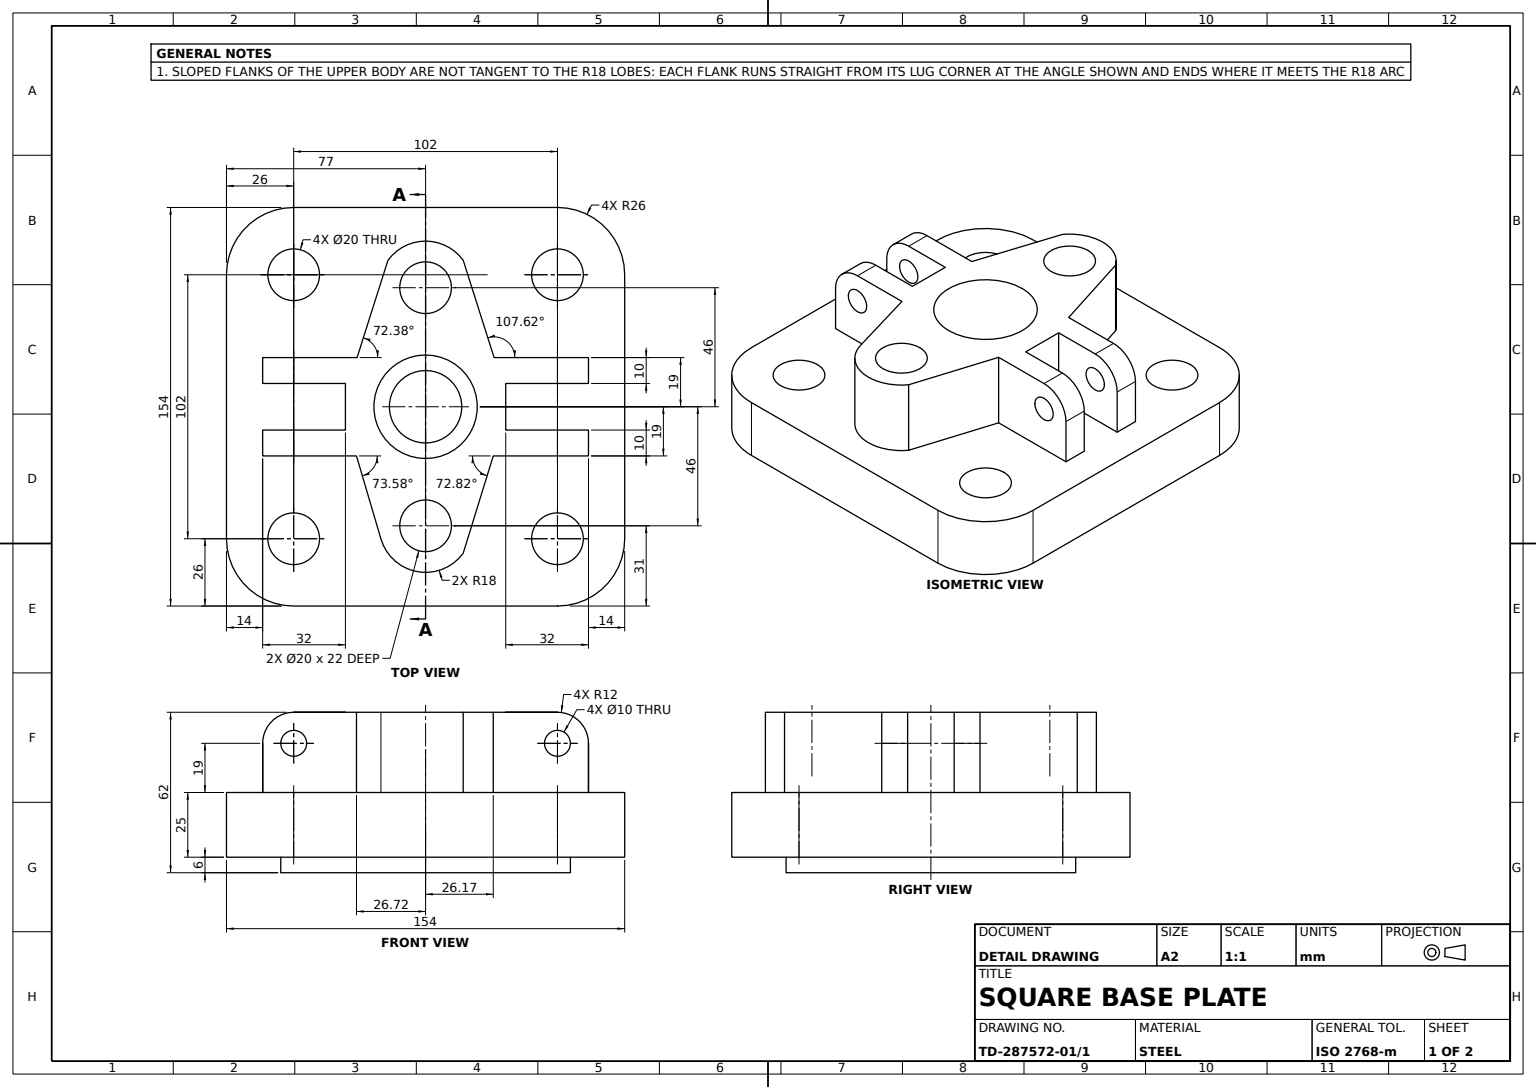
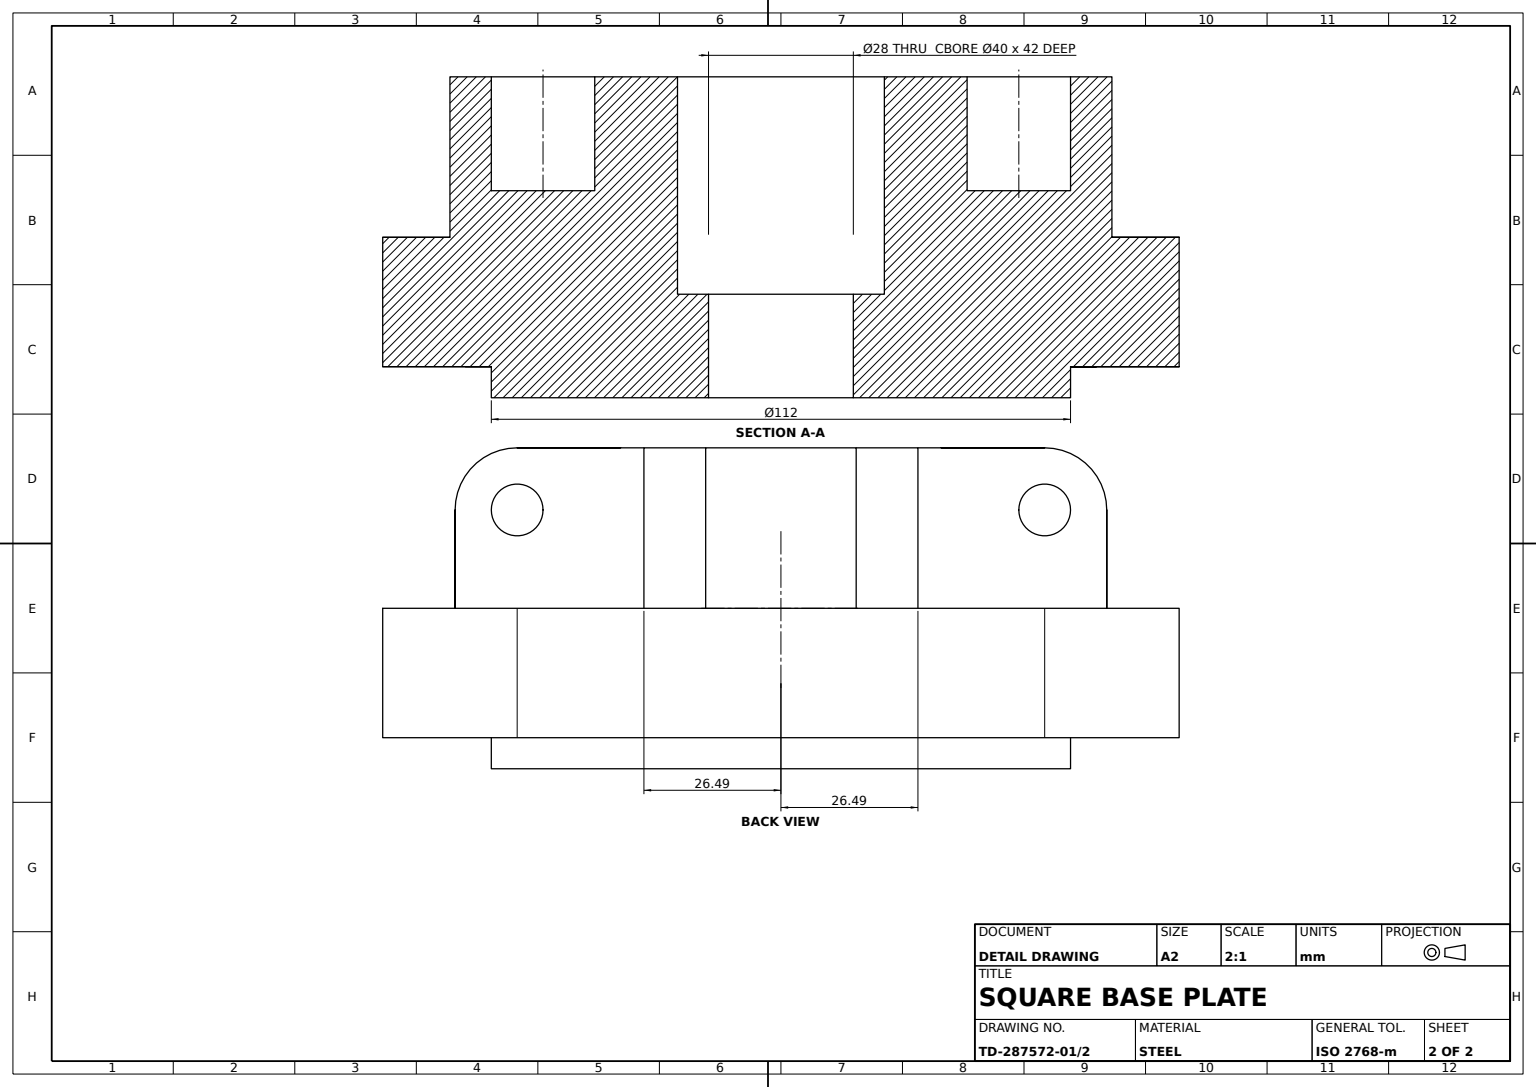
solid
v1 (-63,25,9)
v2 (-31,25,9)
e1 v1 v2 LINE
v3 (-63,44,9)
e2 v1 v3 LINE
v4 (-51,56,9)
e3 v3 v4 CIRCLE(AX(P(-51,44,9),D(0,0,-1),D(1,0,0)),12)
v5 (-31,56,9)
e4 v4 v5 LINE
e5 v2 v5 LINE
v6 (-46,44,9)
v7 (-56,44,9)
e6 v6 v7 CIRCLE(AX(P(-51,44,9),D(0,0,1),D(1,0,0)),5)
e7 v7 v6 CIRCLE(AX(P(-51,44,9),D(0,0,1),D(1,0,0)),5)
face PLANE(AX(P(0,25,9),D(0,0,1),D(1,0,0))) rev [-e1 e2 e3 e4 -e5] [e6 e7]
v8 (0,25,-64)
v9 (-14.551173,25,-56.595441)
e8 v8 v9 CIRCLE(AX(P(0,25,-46),D(0,1,0),D(0,0,1)),18)
v10 (-14.551173,56,-56.595441)
e9 v10 v9 LINE
v11 (0,56,-64)
e10 v11 v10 CIRCLE(AX(P(0,56,-46),D(0,1,0),D(0,0,1)),18)
e11 v11 v8 LINE
face CYL(AX(P(0,56,-46),D(0,-1,0),D(0,0,-1)),18) [e8 -e9 -e10 e11]
v12 (14.551173,56,56.595441)
v13 (14.551173,25,56.595441)
e12 v12 v13 LINE
v14 (-17.266235,56,51.086957)
e13 v14 v12 CIRCLE(AX(P(0,56,46),D(0,1,0),D(0,0,1)),18)
v15 (-17.266235,25,51.086957)
e14 v14 v15 LINE
e15 v15 v13 CIRCLE(AX(P(0,25,46),D(0,1,0),D(0,0,1)),18)
face CYL(AX(P(0,56,46),D(0,-1,0),D(0,0,-1)),18) [-e12 -e13 e14 e15]
v16 (-46,44,19)
v17 (-56,44,19)
e16 v16 v17 CIRCLE(AX(P(-51,44,19),D(0,0,1),D(1,0,0)),5)
e17 v7 v17 LINE
e18 v6 v16 LINE
face CYL(AX(P(-51,44,-99),D(0,0,1),D(1,0,0)),5) rev [e16 -e17 -e6 e18]
v18 (51,0,-61)
v19 (51,25,-61)
e19 v18 v19 LINE
v20 (51,25,-41)
e20 v19 v20 CIRCLE(AX(P(51,25,-51),D(0,1,0),D(0,0,1)),10)
v21 (51,0,-41)
e21 v21 v20 LINE
e22 v18 v21 CIRCLE(AX(P(51,0,-51),D(0,1,0),D(0,0,1)),10)
face CYL(AX(P(51,-87,-51),D(0,1,0),D(0,0,1)),10) rev [e19 e20 -e21 -e22]
v22 (63,44,9)
v23 (63,44,19)
e23 v22 v23 LINE
v24 (51,56,9)
e24 v24 v22 CIRCLE(AX(P(51,44,9),D(0,0,-1),D(-1,0,0)),12)
v25 (51,56,19)
e25 v25 v24 LINE
e26 v23 v25 CIRCLE(AX(P(51,44,19),D(0,0,1),D(1,0,0)),12)
face CYL(AX(P(51,44,-46),D(0,0,-1),D(-1,0,0)),12) [-e23 -e24 -e25 -e26]
v26 (-46,44,-19)
v27 (-56,44,-19)
e27 v26 v27 CIRCLE(AX(P(-51,44,-19),D(0,0,-1),D(-1,0,0)),5)
e28 v27 v26 CIRCLE(AX(P(-51,44,-19),D(0,0,-1),D(-1,0,0)),5)
v28 (-26.491517,25,-19)
v29 (-63,25,-19)
e29 v28 v29 LINE
v30 (-63,44,-19)
e30 v29 v30 LINE
v31 (-51,56,-19)
e31 v30 v31 CIRCLE(AX(P(-51,44,-19),D(0,0,-1),D(-1,0,0)),12)
v32 (-26.491517,56,-19)
e32 v32 v31 LINE
e33 v28 v32 LINE
face PLANE(AX(P(0,25,-19),D(0,0,-1),D(-1,0,0))) [-e27 -e28] [e29 e30 e31 -e32 -e33]
v33 (51,25,41)
v34 (51,25,61)
e34 v33 v34 CIRCLE(AX(P(51,25,51),D(0,1,0),D(0,0,1)),10)
v35 (51,0,61)
e35 v35 v34 LINE
v36 (51,0,41)
e36 v36 v35 CIRCLE(AX(P(51,0,51),D(0,1,0),D(0,0,1)),10)
e37 v36 v33 LINE
face CYL(AX(P(51,-87,51),D(0,1,0),D(0,0,1)),10) rev [e34 -e35 -e36 e37]
v37 (31,25,-9)
v38 (31,25,9)
e38 v37 v38 LINE
v39 (31,56,-9)
e39 v37 v39 LINE
v40 (31,56,9)
e40 v39 v40 LINE
e41 v38 v40 LINE
face PLANE(AX(P(31,25,0),D(-1,0,0),D(0,0,1))) rev [-e38 e39 e40 -e41]
v41 (-31,25,-9)
e42 v41 v2 LINE
v42 (-31,56,-9)
e43 v42 v5 LINE
e44 v41 v42 LINE
face PLANE(AX(P(-31,25,0),D(-1,0,0),D(0,0,1))) [e42 e5 -e43 -e44]
v43 (26.491517,25,-19)
v44 (63,25,-19)
e45 v43 v44 LINE
v45 (26.491517,56,-19)
e46 v43 v45 LINE
v46 (51,56,-19)
e47 v45 v46 LINE
v47 (63,44,-19)
e48 v46 v47 CIRCLE(AX(P(51,44,-19),D(0,0,-1),D(1,0,0)),12)
e49 v44 v47 LINE
v48 (46,44,-19)
v49 (56,44,-19)
e50 v48 v49 CIRCLE(AX(P(51,44,-19),D(0,0,1),D(1,0,0)),5)
e51 v49 v48 CIRCLE(AX(P(51,44,-19),D(0,0,1),D(1,0,0)),5)
face PLANE(AX(P(0,25,-19),D(0,0,1),D(1,0,0))) rev [-e45 e46 e47 e48 -e49] [e50 e51]
e52 v24 v40 LINE
v50 (63,25,9)
e53 v50 v22 LINE
e54 v50 v38 LINE
v51 (56,44,9)
v52 (46,44,9)
e55 v51 v52 CIRCLE(AX(P(51,44,9),D(0,0,-1),D(-1,0,0)),5)
e56 v52 v51 CIRCLE(AX(P(51,44,9),D(0,0,-1),D(-1,0,0)),5)
face PLANE(AX(P(0,25,9),D(0,0,-1),D(-1,0,0))) [-e52 e24 -e53 e54 e41] [-e55 -e56]
v53 (63,25,-9)
e57 v44 v53 LINE
v54 (63,44,-9)
e58 v47 v54 LINE
e59 v53 v54 LINE
face PLANE(AX(P(63,25,0),D(-1,0,0),D(0,0,1))) rev [-e57 e49 e58 -e59]
v55 (-46,44,-9)
e60 v26 v55 LINE
v56 (-56,44,-9)
e61 v55 v56 CIRCLE(AX(P(-51,44,-9),D(0,0,1),D(1,0,0)),5)
e62 v27 v56 LINE
face CYL(AX(P(-51,44,-99),D(0,0,1),D(1,0,0)),5) rev [e60 e61 -e62 e28]
v57 (77,0,-51)
v58 (51,0,-77)
e63 v57 v58 CIRCLE(AX(P(51,0,-51),D(0,1,0),D(0,0,1)),26)
v59 (77,0,51)
e64 v59 v57 LINE
v60 (51,0,77)
e65 v60 v59 CIRCLE(AX(P(51,0,51),D(0,1,0),D(0,0,1)),26)
v61 (-51,0,77)
e66 v61 v60 LINE
v62 (-77,0,51)
e67 v62 v61 CIRCLE(AX(P(-51,0,51),D(0,1,0),D(0,0,1)),26)
v63 (-77,0,-51)
e68 v63 v62 LINE
v64 (-51,0,-77)
e69 v64 v63 CIRCLE(AX(P(-51,0,-51),D(0,1,0),D(0,0,1)),26)
e70 v58 v64 LINE
e71 v35 v36 CIRCLE(AX(P(51,0,51),D(0,1,0),D(0,0,1)),10)
v65 (-51,0,41)
v66 (-51,0,61)
e72 v65 v66 CIRCLE(AX(P(-51,0,51),D(0,1,0),D(0,0,1)),10)
e73 v66 v65 CIRCLE(AX(P(-51,0,51),D(0,1,0),D(0,0,1)),10)
e74 v21 v18 CIRCLE(AX(P(51,0,-51),D(0,1,0),D(0,0,1)),10)
v67 (-51,0,-41)
v68 (-51,0,-61)
e75 v67 v68 CIRCLE(AX(P(-51,0,-51),D(0,1,0),D(0,0,1)),10)
e76 v68 v67 CIRCLE(AX(P(-51,0,-51),D(0,1,0),D(0,0,1)),10)
v69 (0,0,56)
v70 (0,0,-56)
e77 v69 v70 CIRCLE(AX(P(0,0,0),D(0,-1,0),D(0,0,-1)),56)
e78 v70 v69 CIRCLE(AX(P(0,0,0),D(0,-1,0),D(0,0,-1)),56)
face PLANE(AX(P(51,0,51),D(0,1,0),D(0,0,1))) rev [-e63 -e64 -e65 -e66 -e67 -e68 -e69 -e70] [e36 e71] [e72 e73] [e74 e22] [e75 e76] [-e77 -e78]
e79 v10 v32 LINE
e80 v9 v28 LINE
face PLANE(AX(P(-14.551173,56,-56.595441),D(0.953085629,0,0.302700815),D(0.302700815,0,-0.953085629))) rev [-e79 e9 e80 e33]
v71 (51,25,-77)
e81 v71 v58 LINE
v72 (77,25,-51)
e82 v72 v71 CIRCLE(AX(P(51,25,-51),D(0,1,0),D(0,0,1)),26)
e83 v72 v57 LINE
face CYL(AX(P(51,25,-51),D(0,-1,0),D(0,0,-1)),26) [-e81 -e82 e83 e63]
v73 (0,-6,14)
v74 (0,-6,-14)
e84 v73 v74 CIRCLE(AX(P(0,-6,0),D(0,-1,0),D(0,0,-1)),14)
v75 (0,14,-14)
e85 v74 v75 LINE
v76 (0,14,14)
e86 v76 v75 CIRCLE(AX(P(0,14,0),D(0,-1,0),D(0,0,1)),14)
e87 v73 v76 LINE
face CYL(AX(P(0,-62,0),D(0,1,0),D(0,0,1)),14) rev [e84 e85 -e86 -e87]
e88 v34 v33 CIRCLE(AX(P(51,25,51),D(0,1,0),D(0,0,1)),10)
face CYL(AX(P(51,-87,51),D(0,1,0),D(0,0,1)),10) rev [-e37 -e71 e35 e88]
v77 (-51,56,19)
e89 v4 v77 LINE
v78 (-63,44,19)
e90 v78 v3 LINE
e91 v77 v78 CIRCLE(AX(P(-51,44,19),D(0,0,1),D(-1,0,0)),12)
face CYL(AX(P(-51,44,0),D(0,0,1),D(1,0,0)),12) [-e89 -e3 -e90 -e91]
v79 (14.551173,56,-56.595441)
e92 v45 v79 LINE
v80 (14.551173,25,-56.595441)
e93 v43 v80 LINE
e94 v79 v80 LINE
face PLANE(AX(P(14.551173,56,-56.595441),D(-0.953085629,0,0.302700815),D(0.302700815,0,0.953085629))) rev [-e92 -e46 e93 -e94]
e95 v20 v19 CIRCLE(AX(P(51,25,-51),D(0,1,0),D(0,0,1)),10)
face CYL(AX(P(51,-87,-51),D(0,1,0),D(0,0,1)),10) rev [e21 e95 -e19 -e74]
v81 (0,-6,-56)
e96 v81 v70 LINE
v82 (0,-6,56)
e97 v82 v69 LINE
e98 v81 v82 CIRCLE(AX(P(0,-6,0),D(0,-1,0),D(0,0,-1)),56)
face CYL(AX(P(0,-6,0),D(0,1,0),D(0,0,1)),56) [e96 e78 -e97 -e98]
v83 (63,25,19)
e99 v83 v23 LINE
e100 v83 v50 LINE
face PLANE(AX(P(63,25,0),D(1,0,0),D(0,0,-1))) [-e99 e100 e53 e23]
v84 (-51,25,61)
v85 (-51,25,41)
e101 v84 v85 CIRCLE(AX(P(-51,25,51),D(0,1,0),D(0,0,1)),10)
e102 v65 v85 LINE
e103 v66 v84 LINE
face CYL(AX(P(-51,-87,51),D(0,1,0),D(0,0,1)),10) rev [e101 -e102 -e73 e103]
e104 v17 v16 CIRCLE(AX(P(-51,44,19),D(0,0,1),D(1,0,0)),5)
v86 (-63,25,19)
e105 v86 v78 LINE
v87 (-26.719654,25,19)
e106 v87 v86 LINE
v88 (-26.719654,56,19)
e107 v87 v88 LINE
e108 v88 v77 LINE
face PLANE(AX(P(0,25,19),D(0,0,-1),D(-1,0,0))) rev [-e16 -e104] [-e105 -e106 e107 e108 e91]
e109 v56 v55 CIRCLE(AX(P(-51,44,-9),D(0,0,1),D(1,0,0)),5)
face CYL(AX(P(-51,44,-99),D(0,0,1),D(1,0,0)),5) rev [-e60 e27 e62 e109]
e110 v88 v14 LINE
e111 v87 v15 LINE
face PLANE(AX(P(-29.736294,56,8.76087),D(0.959235281,0,-0.282608696),D(-0.282608696,0,-0.959235281))) rev [-e110 -e107 e111 -e14]
e112 v85 v84 CIRCLE(AX(P(-51,25,51),D(0,1,0),D(0,0,1)),10)
face CYL(AX(P(-51,-87,51),D(0,1,0),D(0,0,1)),10) rev [e112 -e103 -e72 e102]
v89 (0,14,-20)
v90 (0,14,20)
e113 v89 v90 CIRCLE(AX(P(0,14,0),D(0,1,0),D(0,0,1)),20)
v91 (0,56,-20)
e114 v89 v91 LINE
v92 (0,56,20)
e115 v91 v92 CIRCLE(AX(P(0,56,0),D(0,1,0),D(0,0,1)),20)
e116 v90 v92 LINE
face CYL(AX(P(0,14,0),D(0,1,0),D(0,0,1)),20) rev [-e113 e114 e115 -e116]
v93 (51,56,-9)
e117 v54 v93 CIRCLE(AX(P(51,44,-9),D(0,0,1),D(-1,0,0)),12)
e118 v93 v46 LINE
face CYL(AX(P(51,44,0),D(0,0,-1),D(-1,0,0)),12) [-e117 -e58 -e48 -e118]
v94 (0,56,-56)
v95 (0,56,-36)
e119 v94 v95 CIRCLE(AX(P(0,56,-46),D(0,1,0),D(0,0,1)),10)
v96 (0,34,-36)
e120 v96 v95 LINE
v97 (0,34,-56)
e121 v97 v96 CIRCLE(AX(P(0,34,-46),D(0,1,0),D(0,0,1)),10)
e122 v97 v94 LINE
face CYL(AX(P(0,34,-46),D(0,1,0),D(0,0,1)),10) rev [e119 -e120 -e121 e122]
v98 (46,44,19)
v99 (56,44,19)
e123 v98 v99 CIRCLE(AX(P(51,44,19),D(0,0,1),D(1,0,0)),5)
e124 v51 v99 LINE
e125 v52 v98 LINE
face CYL(AX(P(51,44,-99),D(0,0,1),D(1,0,0)),5) rev [e123 -e124 e55 e125]
e126 v92 v91 CIRCLE(AX(P(0,56,0),D(0,1,0),D(0,0,1)),20)
e127 v90 v89 CIRCLE(AX(P(0,14,0),D(0,1,0),D(0,0,1)),20)
face CYL(AX(P(0,14,0),D(0,1,0),D(0,0,1)),20) rev [e116 e126 -e114 -e127]
v100 (-51,56,-9)
e128 v31 v100 LINE
v101 (-63,44,-9)
e129 v101 v30 LINE
e130 v100 v101 CIRCLE(AX(P(-51,44,-9),D(0,0,1),D(1,0,0)),12)
face CYL(AX(P(-51,44,-46),D(0,0,1),D(1,0,0)),12) [-e128 -e31 -e129 -e130]
v102 (77,25,51)
e131 v102 v72 LINE
e132 v102 v59 LINE
face PLANE(AX(P(77,25,0),D(-1,0,0),D(0,0,1))) rev [e64 -e83 -e131 e132]
v103 (0,34,56)
v104 (0,56,56)
e133 v103 v104 LINE
v105 (0,34,36)
e134 v105 v103 CIRCLE(AX(P(0,34,46),D(0,1,0),D(0,0,1)),10)
v106 (0,56,36)
e135 v105 v106 LINE
e136 v106 v104 CIRCLE(AX(P(0,56,46),D(0,1,0),D(0,0,1)),10)
face CYL(AX(P(0,34,46),D(0,1,0),D(0,0,1)),10) rev [-e133 -e134 e135 e136]
e137 v80 v8 CIRCLE(AX(P(0,25,-46),D(0,1,0),D(0,0,1)),18)
e138 v79 v11 CIRCLE(AX(P(0,56,-46),D(0,1,0),D(0,0,1)),18)
face CYL(AX(P(0,56,-46),D(0,-1,0),D(0,0,-1)),18) [e137 -e11 -e138 e94]
v107 (-77,25,-51)
v108 (-77,25,51)
e139 v107 v108 LINE
e140 v107 v63 LINE
e141 v108 v62 LINE
face PLANE(AX(P(-77,25,-51),D(1,0,0),D(0,0,-1))) rev [-e139 e140 e68 -e141]
v109 (-51,25,-41)
e142 v67 v109 LINE
v110 (-51,25,-61)
e143 v109 v110 CIRCLE(AX(P(-51,25,-51),D(0,1,0),D(0,0,1)),10)
e144 v68 v110 LINE
face CYL(AX(P(-51,-87,-51),D(0,1,0),D(0,0,1)),10) rev [e142 e143 -e144 -e75]
e145 v96 v97 CIRCLE(AX(P(0,34,-46),D(0,1,0),D(0,0,1)),10)
face PLANE(AX(P(0,34,-46),D(0,1,0),D(0,0,1))) [e121 e145]
e146 v99 v98 CIRCLE(AX(P(51,44,19),D(0,0,1),D(1,0,0)),5)
face CYL(AX(P(51,44,-99),D(0,0,1),D(1,0,0)),5) rev [e56 e124 e146 -e125]
face CYL(AX(P(-51,44,-99),D(0,0,1),D(1,0,0)),5) rev [-e18 -e7 e17 e104]
v111 (-51,25,-77)
e147 v111 v64 LINE
e148 v71 v111 LINE
face PLANE(AX(P(51,25,-77),D(0,0,1),D(1,0,0))) rev [e70 -e147 -e148 e81]
e149 v111 v107 CIRCLE(AX(P(-51,25,-51),D(0,1,0),D(0,0,1)),26)
face CYL(AX(P(-51,25,-51),D(0,-1,0),D(0,0,-1)),26) [e69 -e140 -e149 e147]
v112 (46,44,-9)
e150 v48 v112 LINE
v113 (56,44,-9)
e151 v113 v112 CIRCLE(AX(P(51,44,-9),D(0,0,-1),D(-1,0,0)),5)
e152 v49 v113 LINE
face CYL(AX(P(51,44,-99),D(0,0,1),D(1,0,0)),5) rev [-e50 e150 -e151 -e152]
v114 (51,25,77)
e153 v114 v102 CIRCLE(AX(P(51,25,51),D(0,1,0),D(0,0,1)),26)
e154 v114 v60 LINE
face CYL(AX(P(51,25,51),D(0,-1,0),D(0,0,-1)),26) [-e153 e154 e65 -e132]
e155 v112 v113 CIRCLE(AX(P(51,44,-9),D(0,0,-1),D(-1,0,0)),5)
face CYL(AX(P(51,44,-99),D(0,0,1),D(1,0,0)),5) rev [-e150 -e51 e152 -e155]
e156 v95 v94 CIRCLE(AX(P(0,56,-46),D(0,1,0),D(0,0,1)),10)
face CYL(AX(P(0,34,-46),D(0,1,0),D(0,0,1)),10) rev [e156 -e122 -e145 e120]
e157 v86 v1 LINE
face PLANE(AX(P(-63,25,0),D(1,0,0),D(0,0,-1))) rev [e90 -e2 -e157 e105]
v115 (-63,25,-9)
e158 v29 v115 LINE
e159 v115 v101 LINE
face PLANE(AX(P(-63,25,0),D(-1,0,0),D(0,0,1))) [-e30 e158 e159 e129]
v116 (26.17373,56,19)
e160 v12 v116 LINE
e161 v116 v25 LINE
e162 v93 v39 LINE
e163 v100 v42 LINE
e164 v104 v106 CIRCLE(AX(P(0,56,46),D(0,1,0),D(0,0,1)),10)
face PLANE(AX(P(0,56,-46),D(0,1,0),D(0,0,1))) [e160 e161 e25 e52 -e40 -e162 e118 -e47 e92 e138 e10 e79 e32 e128 e163 e43 -e4 e89 -e108 e110 e13] [-e136 -e164] [-e126 -e115] [-e119 -e156]
v117 (-51,25,77)
e165 v108 v117 CIRCLE(AX(P(-51,25,51),D(0,1,0),D(0,0,1)),26)
e166 v117 v114 LINE
v118 (26.17373,25,19)
e167 v118 v83 LINE
e168 v13 v118 LINE
e169 v115 v41 LINE
e170 v53 v37 LINE
e171 v110 v109 CIRCLE(AX(P(-51,25,-51),D(0,1,0),D(0,0,1)),10)
face PLANE(AX(P(51,25,51),D(0,1,0),D(0,0,1))) [-e101 -e112] [-e95 -e20] [e82 e148 e149 e139 e165 e166 e153 e131] [-e54 -e100 -e167 -e168 -e15 -e111 e106 e157 e1 -e42 -e169 -e158 -e29 -e80 -e8 -e137 -e93 e45 e57 e170 e38] [-e143 -e171] [-e34 -e88]
e172 v118 v116 LINE
face PLANE(AX(P(0,25,19),D(0,0,1),D(1,0,0))) [-e161 -e172 e167 e99 e26] [-e146 -e123]
e173 v103 v105 CIRCLE(AX(P(0,34,46),D(0,1,0),D(0,0,1)),10)
face CYL(AX(P(0,34,46),D(0,1,0),D(0,0,1)),10) rev [e133 e164 -e135 -e173]
e174 v82 v81 CIRCLE(AX(P(0,-6,0),D(0,-1,0),D(0,0,-1)),56)
face CYL(AX(P(0,-6,0),D(0,1,0),D(0,0,1)),56) [e77 -e96 -e174 e97]
e175 v75 v76 CIRCLE(AX(P(0,14,0),D(0,-1,0),D(0,0,1)),14)
face PLANE(AX(P(0,14,0),D(0,1,0),D(0,0,1))) [e113 e127] [e175 e86]
face PLANE(AX(P(0,25,-9),D(0,0,1),D(1,0,0))) [-e109 -e61] [e44 -e163 e130 -e159 e169]
face CYL(AX(P(-51,-87,-51),D(0,1,0),D(0,0,1)),10) rev [-e76 e144 e171 -e142]
e176 v74 v73 CIRCLE(AX(P(0,-6,0),D(0,-1,0),D(0,0,-1)),14)
face PLANE(AX(P(0,-6,0),D(0,-1,0),D(0,0,-1))) [e174 e98] [-e84 -e176]
face PLANE(AX(P(0,34,46),D(0,1,0),D(0,0,1))) [e173 e134]
face CYL(AX(P(0,-62,0),D(0,1,0),D(0,0,1)),14) rev [e87 -e175 -e85 e176]
e177 v117 v61 LINE
face PLANE(AX(P(-51,25,77),D(0,0,-1),D(-1,0,0))) rev [-e154 -e166 e177 e66]
face PLANE(AX(P(14.551173,56,56.595441),D(-0.955387242,0,-0.295356087),D(-0.295356087,0,0.955387242))) rev [-e160 e12 e168 e172]
face PLANE(AX(P(0,25,-9),D(0,0,-1),D(-1,0,0))) rev [e151 e155] [-e39 -e170 e59 e117 e162]
face CYL(AX(P(-51,25,51),D(0,-1,0),D(0,0,-1)),26) [e67 -e177 -e165 e141]
